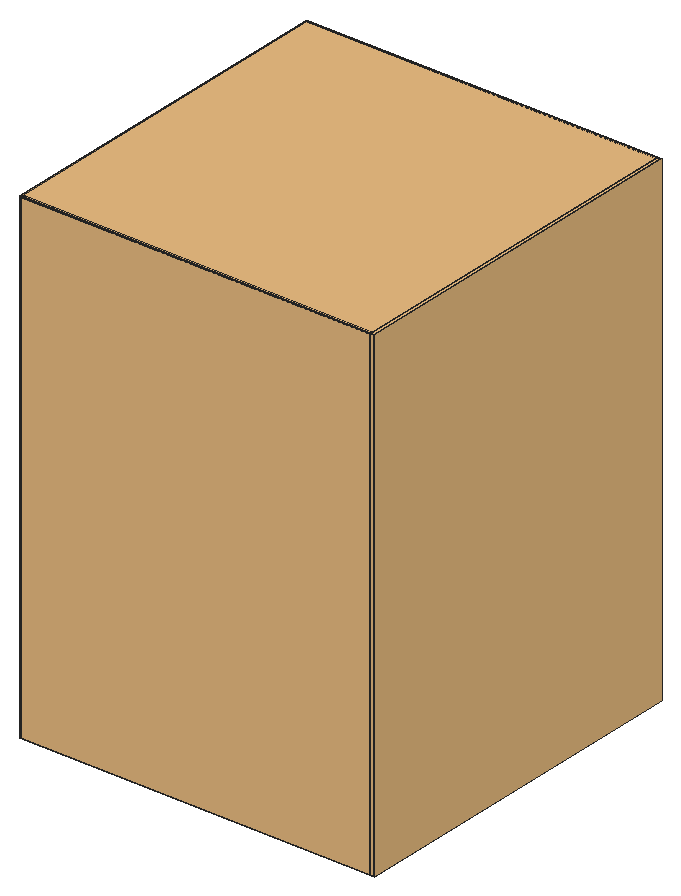
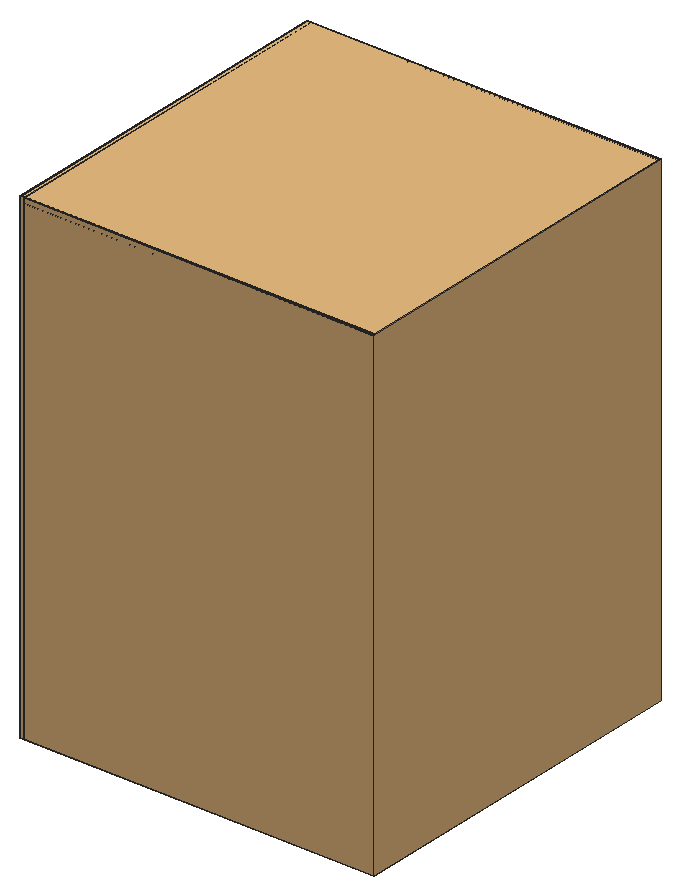
# SketchUp Ruby script. Lengths in inches.
U = 1.inch
M = Sketchup.active_model
def pt(a) = Geom::Point3d.new(a.map { |v| v * U })
def face(e, loops, mat)
  f = e.add_face(loops[0].map { |a| pt(a) })
  loops[1..].each { |l| e.add_face(l.map { |a| pt(a) }).erase! }
  f.material = f.back_material = mat if mat
  f
end
# faces: each face lists its corners as indices into pts; further lists are holes
def faces(e, pts, list, mat = nil) = list.each { |f| face(e, (f[0].is_a?(Array) ? f : [f]).map { |l| l.map { |i| pts[i] } }, mat) }
# xy, xz, yz: faces in a plane at the given z, y or x. An outline is a flat list of corners, or four numbers for a rectangle; further outlines are holes
def ring(l) = l.size == 4 ? [[l[0], l[1]], [l[2], l[1]], [l[2], l[3]], [l[0], l[3]]] : l.each_slice(2).to_a
def flat(e, list, mat, &to3) = list.each { |f| face(e, (f[0].is_a?(Array) ? f : [f]).map { |l| ring(l).map { |u, v| to3.(u, v) } }, mat) }
def xy(e, z, list, mat = nil) = flat(e, list, mat) { |x, y| [x, y, z] }
def xz(e, y, list, mat = nil) = flat(e, list, mat) { |x, z| [x, y, z] }
def yz(e, x, list, mat = nil) = flat(e, list, mat) { |y, z| [x, y, z] }
def lines(e, pts, list) = list.each { |a, b| e.add_line(pt(pts[a]), pt(pts[b])) }
# prism: a flat outline (further loops are holes) pulled along v
def prism(e, loops, v, mat = nil)
  f = face(e, loops, mat); d = Geom::Vector3d.new(v.map { |x| x * U })
  f.pushpull(f.normal.samedirection?(d) ? d.length : -d.length)
end
def box(e, o, s, mat = nil) = prism(e, [[o, [o[0] + s[0], o[1], o[2]], [o[0] + s[0], o[1] + s[1], o[2]], [o[0], o[1] + s[1], o[2]]]], [0, 0, s[2]], mat)
def at(x, y, z, deg = 0) = Geom::Transformation.translation(pt([x, y, z])) * Geom::Transformation.rotation(ORIGIN, Z_AXIS, deg.degrees)
def axes(o, x, y, z) = Geom::Transformation.new([*x, 0, *y, 0, *z, 0, *pt(o).to_a, 1])
def part(name) = M.definitions.add(name)
# library, detail: a bought-in or finely detailed component or shape, given as its bounding box
def library(name, o, s) = part(name).tap { |d| box(d.entities, o, s) }
def detail(e, o, s) = box(e.add_group.entities, o, s)
def put(e, d, t, mat = nil) = e.add_instance(d, t).tap { |i| i.material = mat if mat }
def group(e, t, mat = nil) = e.add_group.tap { |g| g.transformation = t; g.material = mat if mat }.entities
root = M.entities
M.materials.add("green").color = [174, 139, 102]
M.materials.add("vio").color = [206, 114, 100]
c1 = part("3DGeom~220_Defintion")
p = [[-57.64,36.25,-500],[-74.66,-181.39,-451.57],[-284.21,-169.14,-366.97],[199.77,12.4,-463.71],[-284.21,-169.14,-366.97],[-299.61,50.39,-402.32],
  [197.74,223.52,-383.03],[-25.18,244.18,-414.46],[-299.61,50.39,-402.32],[-25.18,244.18,-414.46],[148.26,-202.04,-420.14],[403.65,-14.77,-303.17],
  [374.3125,199.99,-244],[374.3125,199.99,-244],[-71.68,-350.42,-282.14],[-192.66,-343.35,-233.3],[-192.66,-343.35,-233.3],[-284.21,-169.14,-366.97],
  [57.03,-362.35,-264],[324.83,-225.57,-281.11],[-25.18,244.18,-414.46],[-299.61,50.39,-402.32],[-234.73,256.42,-329.86],[142.74,374.75,-199.71],
  [-25.18,244.18,-414.46],[14.03,386.67,-217.86],[-25.18,244.18,-414.46],[-234.73,256.42,-329.86],[142.74,374.75,-199.71],[-25.18,244.18,-414.46],
  [14.03,386.67,-217.86],[-299.61,50.39,-402.32],[-284.21,-169.14,-366.97],[-424.23,-168.6,-189.02],[-461.29,51.02,-196.83],[-234.73,256.42,-329.86],
  [244.68,361.16,-119.44],[374.3125,199.99,-244],[197.74,223.52,-383.03],[197.74,223.52,-383.03],[142.74,374.75,-199.71],[-192.66,-343.35,-233.3],
  [-273.5,-343.04,-130.56],[-234.73,256.42,-329.86],[-374.75,256.97,-151.9],[-106.95,393.74,-169.02],[-374.75,256.97,-151.9],[499.375,-37.98,-61.39],
  [324.83,-225.57,-281.11],[403.65,-14.77,-303.17],[457.21,179.89,-34.61],[403.65,-14.77,-303.17],[403.65,-14.77,-303.17],[374.3125,199.99,-244],
  [-192.66,-343.35,-233.3],[-71.68,-350.42,-282.14],[-49.48,-425.5625,-37.11],[-71.68,-350.42,-282.14],[57.03,-362.35,-264],[158.97,-375.93,-183.73],
  [407.73,-245.68,-71.73],[158.97,-375.93,-183.73],[324.83,-225.57,-281.11],[407.73,-245.68,-71.73],[324.83,-225.57,-281.11],[57.03,-362.35,-264],
  [158.97,-375.93,-183.73],[292.54,349.56,1.44],[374.3125,199.99,-244],[292.54,349.56,1.44],[374.3125,199.99,-244],[244.68,361.16,-119.44],
  [-273.5,-343.04,-130.56],[-192.66,-343.35,-233.3],[49.48,425.5625,37.11],[-457.21,-179.89,34.61],[-499.375,37.98,61.39],[-374.75,256.97,-151.9],
  [-292.54,-349.56,-1.44],[158.97,-375.93,-183.73],[206.83,-387.54,-62.84],[407.73,-245.68,-71.73],[158.97,-375.93,-183.73],[-187.79,394.06,-66.27],
  [-374.75,256.97,-151.9],[-407.73,245.68,71.73],[-407.73,245.68,71.73],[-292.54,-349.56,-1.44],[-273.5,-343.04,-130.56],[292.54,349.56,1.44],
  [374.75,-256.97,151.9],[407.73,-245.68,-71.73],[461.29,-51.02,196.83],[374.75,-256.97,151.9],[-206.83,387.54,62.84],[187.79,-394.06,66.27],
  [374.75,-256.97,151.9],[424.23,168.6,189.02],[-244.68,-361.16,119.44],[-292.54,-349.56,-1.44],[-142.74,-374.75,199.71],[-14.03,-386.67,217.86],
  [106.95,-393.74,169.02],[273.5,343.04,130.56],[273.5,343.04,130.56],[292.54,349.56,1.44],[-244.68,-361.16,119.44],[273.5,343.04,130.56],
  [-244.68,-361.16,119.44],[-374.3125,-199.99,244],[-374.3125,-199.99,244],[192.66,343.35,233.3],[71.68,350.42,282.14],[-57.03,362.35,264],
  [-158.97,375.93,183.73],[-374.3125,-199.99,244],[-403.65,14.77,303.17],[-407.73,245.68,71.73],[-403.65,14.77,303.17],[-324.83,225.57,281.11],
  [-324.83,225.57,281.11],[234.73,-256.42,329.86],[234.73,-256.42,329.86],[374.75,-256.97,151.9],[-407.73,245.68,71.73],[-403.65,14.77,303.17],
  [-324.83,225.57,281.11],[-374.3125,-199.99,244],[192.66,343.35,233.3],[273.5,343.04,130.56],[299.61,-50.39,402.32],[234.73,-256.42,329.86],
  [25.18,-244.18,414.46],[25.18,-244.18,414.46],[234.73,-256.42,329.86],[-158.97,375.93,183.73],[-324.83,225.57,281.11],[-148.26,202.04,420.14],
  [-158.97,375.93,183.73],[-57.03,362.35,264],[284.21,169.14,366.97],[192.66,343.35,233.3],[-197.74,-223.52,383.03],[-142.74,-374.75,199.71],
  [-14.03,-386.67,217.86],[-374.3125,-199.99,244],[-197.74,-223.52,383.03],[-14.03,-386.67,217.86],[25.18,-244.18,414.46],[71.68,350.42,282.14],
  [284.21,169.14,366.97],[192.66,343.35,233.3],[-403.65,14.77,303.17],[-374.3125,-199.99,244],[-57.03,362.35,264],[74.66,181.39,451.57],
  [-57.03,362.35,264],[71.68,350.42,282.14],[-199.77,-12.4,463.71],[71.68,350.42,282.14],[284.21,169.14,366.97],[57.64,-36.25,500],
  [234.73,-256.42,329.86],[234.73,-256.42,329.86],[299.61,-50.39,402.32],[299.61,-50.39,402.32],[284.21,169.14,366.97],[299.61,-50.39,402.32]]
faces(c1.entities,p,[[0,1,2],[3,1,0],[0,4,5],[6,3,0],[7,0,8],[6,0,9],[3,10,1],[11,10,3],
  [12,11,3],[13,3,6],[1,14,15],[10,14,1],[1,16,17],[10,18,14],[19,18,10],[11,19,10],
  [20,21,22],[23,6,24],[25,26,27],[28,29,30],[31,32,33],[31,33,34],[35,31,34],[36,37,38],
  [36,39,40],[32,41,42],[32,42,33],[43,34,44],[45,27,46],[25,27,45],[47,48,49],[50,47,51],
  [50,52,53],[54,55,56],[57,58,56],[19,59,18],[60,61,62],[47,63,64],[65,66,56],[67,50,68],
  [69,70,71],[72,73,56],[40,25,74],[25,45,74],[36,40,74],[34,75,76],[34,33,75],[77,34,76],
  [33,78,75],[33,42,78],[79,80,56],[81,80,82],[45,46,83],[45,83,74],[84,76,85],[83,46,86],
  [87,88,56],[89,36,74],[90,80,91],[92,93,63],[92,63,47],[83,86,94],[83,94,74],[80,95,56],
  [96,95,80],[97,92,47],[97,47,50],[98,99,56],[100,98,56],[101,100,56],[95,102,56],[102,101,56],
  [103,97,50],[104,50,105],[75,78,106],[107,89,74],[75,108,109],[76,75,110],[111,107,74],[112,111,74],
  [113,112,74],[114,113,74],[94,114,74],[76,115,116],[117,76,118],[94,86,119],[94,120,114],[121,102,95],
  [122,95,123],[124,125,126],[127,98,100],[128,97,129],[130,131,93],[130,93,92],[132,101,102],[133,102,134],
  [135,136,137],[138,137,139],[140,92,97],[141,140,97],[140,130,92],[142,143,144],[145,100,146],[142,147,148],
  [149,150,151],[152,153,142],[154,137,155],[156,155,157],[136,152,158],[136,158,137],[159,155,160],[152,142,158],
  [161,148,162],[161,163,164],[155,165,166],[158,142,148],[155,161,167],[158,148,161],[137,158,161],[137,161,155]],"vio")
c2 = library("3DGeom~98_Defintion",[-97.72,-35.49,-500],[195.44,70.98,1000])
c3 = part("3DGeom~99_Defintion")
p = [[97.72,22.79,-497.94],[82.82,12.47,-499.74],[76.21,14.6,-500],[97.72,22.79,-497.94],[76.21,14.6,-500],[71.74,19.25,-499.92],
  [97.72,22.79,-497.94],[71.74,19.25,-499.92],[70.59,25.16,-499.53],[97.72,22.79,-497.94],[89.78,13.42,-499.21],[82.82,12.47,-499.74],
  [97.72,22.79,-497.94],[70.59,25.16,-499.53],[73.07,30.76,-498.92],[97.72,22.79,-497.94],[95.24,17.19,-498.55],[89.78,13.42,-499.21],
  [97.72,22.79,-497.94],[73.07,30.76,-498.92],[78.53,34.54,-498.26],[97.72,22.79,-497.94],[78.53,34.54,-498.26],[85.49,35.49,-497.73],
  [97.72,22.79,-497.94],[85.49,35.49,-497.73],[92.1,33.35,-497.47],[97.72,22.79,-497.94],[92.1,33.35,-497.47],[96.57,28.7,-497.55],
  [-93.36,-33.24,487.31],[-75.65,-25.4,500],[-97.72,-22.56,484.25],[-93.36,-33.24,487.31],[-97.72,-22.56,484.25],[-96.91,-28.5,484.8],
  [-97.72,-22.56,484.25],[-75.65,-25.4,500],[-91.05,-13.3,489.05],[-97.72,-22.56,484.25],[-91.05,-13.3,489.05],[-95.58,-16.99,485.8],
  [-82.33,-34.66,495.19],[-93.36,-33.24,487.31],[-88.02,-35.49,491.12],[-82.33,-34.66,495.19],[-75.65,-25.4,500],[-93.36,-33.24,487.31],
  [-91.05,-13.3,489.05],[-75.65,-25.4,500],[-80.01,-14.72,496.93],[-91.05,-13.3,489.05],[-80.01,-14.72,496.93],[-85.35,-12.47,493.125],
  [-75.65,-25.4,500],[-82.33,-34.66,495.19],[-77.8,-30.96,498.44],[-75.65,-25.4,500],[-76.46,-19.45,499.45],[-80.01,-14.72,496.93]]
faces(c3.entities,p,[[0,1,2],[3,4,5],[6,7,8],[9,10,11],[12,13,14],[15,16,17],[18,19,20],[21,22,23],
  [24,25,26],[27,28,29],[30,31,32],[33,34,35],[36,37,38],[39,40,41],[42,43,44],[45,46,47],
  [48,49,50],[51,52,53],[54,55,56],[57,58,59]],"green")
c4 = part("3DGeom~242_Defintion")
p = [[-230.85,-87.93,-431.85],[22.11,-101.53,-485.51],[16.43,-294.21,-360.73],[264.23,-254.8,-301.01],[16.43,-294.21,-360.73],[269.15,-87.93,-409.08],
  [264.23,-254.8,-301.01],[-231.0625,102.5,-427.26],[21.87,118.36,-480.21],[-230.85,-87.93,-431.85],[268.9375,102.5,-404.49],[-236.35,265.46,-311.23],
  [15.77,306.53,-346.23],[-236.35,265.46,-311.23],[-230.85,-87.93,-431.85],[16.43,-294.21,-360.73],[-235.78,-254.8,-323.78],[-421.96,-50.77,-262.47],
  [-230.85,-87.93,-431.85],[-235.78,-254.8,-323.78],[-422.08,59.18,-259.82],[-230.85,-87.93,-431.85],[-422.08,59.18,-259.82],[-230.85,-87.93,-431.85],
  [-421.96,-50.77,-262.47],[-425.13,153.27,-192.83],[-231.0625,102.5,-427.26],[-422.08,59.18,-259.82],[-236.35,265.46,-311.23],[-231.0625,102.5,-427.26],
  [269.15,-87.93,-409.08],[441.23,-147.11,-160.65],[264.23,-254.8,-301.01],[269.15,-87.93,-409.08],[444.07,-50.76,-223.04],[268.9375,102.5,-404.49],
  [269.15,-87.93,-409.08],[268.9375,102.5,-404.49],[443.95,59.18,-220.39],[263.65,265.47,-288.46],[268.9375,102.5,-404.49],[263.65,265.47,-288.46],
  [-235.78,-254.8,-323.78],[16.43,-294.21,-360.73],[6.34,-408.0625,-139.28],[255.49,-353.39,-109.24],[264.23,-254.8,-301.01],[-245.29,357.3,-114.86],
  [15.77,306.53,-346.23],[-236.35,265.46,-311.23],[5.44,412.57,-119.48],[263.65,265.47,-288.46],[15.77,306.53,-346.23],[-245.29,357.3,-114.86],
  [15.77,306.53,-346.23],[-235.78,-254.8,-323.78],[-244.51,-353.39,-132.01],[-424.8,-147.11,-200.08],[-244.51,-353.39,-132.01],[-430.29,206.29,-79.46],
  [-245.29,357.3,-114.86],[264.23,-254.8,-301.01],[436.18,-204.03,-49.92],[255.49,-353.39,-109.24],[264.23,-254.8,-301.01],[263.65,265.47,-288.46],
  [440.9,153.27,-153.4],[254.71,357.3,-92.09],[263.65,265.47,-288.46],[254.71,357.3,-92.09],[263.65,265.47,-288.46],[-500,0,-22.77],
  [500,0,22.77],[-429.84,-204.03,-89.36],[435.73,206.29,-40.02],[254.71,357.3,-92.09],[-244.51,-353.39,-132.01],[-5.44,-412.57,119.48],
  [245.29,-357.3,114.86],[-244.51,-353.39,-132.01],[-254.71,-357.3,92.09],[-254.71,-357.3,92.09],[-255.49,353.39,109.24],[-6.34,408.0625,139.28],
  [-255.49,353.39,109.24],[-245.29,357.3,-114.86],[-436.18,204.03,49.92],[-255.49,353.39,109.24],[255.49,-353.39,-109.24],[430.29,-206.29,79.46],
  [245.29,-357.3,114.86],[255.49,-353.39,-109.24],[244.51,353.39,132.01],[254.71,357.3,-92.09],[244.51,353.39,132.01],[-435.73,-206.29,40.02],
  [429.84,204.03,89.36],[244.51,353.39,132.01],[-440.9,-153.27,153.4],[-443.95,-59.18,220.39],[-444.07,50.77,223.04],[-441.23,147.11,160.65],
  [425.13,-153.27,192.83],[422.08,-59.18,259.82],[421.96,50.77,262.47],[424.8,147.11,200.08],[-263.65,-265.47,288.46],[245.29,-357.3,114.86],
  [235.78,254.8,323.78],[235.78,254.8,323.78],[244.51,353.39,132.01],[-254.71,-357.3,92.09],[-15.77,-306.53,346.23],[-254.71,-357.3,92.09],
  [-15.77,-306.53,346.23],[-263.65,-265.47,288.46],[-264.22,254.8,301.01],[-264.22,254.8,301.01],[-255.49,353.39,109.24],[236.35,-265.47,311.23],
  [245.29,-357.3,114.86],[236.35,-265.47,311.23],[236.35,-265.47,311.23],[-15.77,-306.53,346.23],[-16.43,294.21,360.73],[235.78,254.8,323.78],
  [-264.22,254.8,301.01],[-268.9375,-102.5,404.49],[236.35,-265.47,311.23],[230.85,87.93,431.85],[230.85,87.93,431.85],[235.78,254.8,323.78],
  [-269.15,87.93,409.08],[236.35,-265.47,311.23],[231.0625,-102.5,427.26],[231.0625,-102.5,427.26],[422.08,-59.18,259.82],[421.96,50.77,262.47],
  [421.96,50.77,262.47],[230.85,87.93,431.85],[-263.65,-265.47,288.46],[-15.77,-306.53,346.23],[-21.87,-118.36,480.21],[-263.65,-265.47,288.46],
  [-268.9375,-102.5,404.49],[-269.15,87.93,409.08],[-16.43,294.21,360.73],[-264.22,254.8,301.01],[236.35,-265.47,311.23],[-22.11,101.53,485.51],
  [235.78,254.8,323.78],[235.78,254.8,323.78],[-16.43,294.21,360.73],[-269.15,87.93,409.08],[-16.43,294.21,360.73],[-268.9375,-102.5,404.49],
  [-268.9375,-102.5,404.49],[-269.15,87.93,409.08]]
faces(c4.entities,p,[[0,1,2],[1,3,4],[1,5,6],[7,8,1],[7,1,9],[8,5,1],[8,10,5],[11,8,7],
  [12,10,8],[13,12,8],[14,15,16],[17,18,19],[20,7,21],[22,23,24],[25,26,27],[25,28,29],
  [30,31,32],[33,34,31],[35,34,36],[37,38,34],[39,38,40],[12,41,10],[42,43,44],[43,45,44],
  [43,46,45],[47,48,49],[50,51,52],[53,50,54],[55,44,56],[57,19,58],[17,19,57],[59,28,25],
  [59,60,28],[61,62,63],[64,31,62],[65,66,38],[67,66,68],[50,69,70],[17,57,71],[27,17,71],
  [25,27,71],[31,34,72],[34,38,72],[38,66,72],[57,58,73],[57,73,71],[59,25,71],[62,31,72],
  [66,74,72],[75,74,66],[76,44,77],[44,78,77],[44,45,78],[79,77,80],[73,58,81],[82,83,50],
  [84,50,85],[83,69,50],[86,87,60],[86,60,59],[88,89,90],[91,62,89],[92,74,93],[83,94,69],
  [73,81,95],[73,95,71],[86,59,71],[89,62,72],[74,96,72],[97,96,74],[95,98,71],[98,99,71],
  [99,100,71],[101,86,71],[100,101,71],[102,89,72],[103,102,72],[104,103,72],[105,104,72],[96,105,72],
  [95,81,106],[95,106,98],[101,87,86],[107,89,102],[108,105,96],[109,96,110],[111,77,112],[113,114,115],
  [101,116,87],[117,83,118],[77,78,119],[120,102,121],[77,122,123],[124,125,94],[124,94,83],[126,124,83],
  [98,106,127],[98,127,99],[100,116,101],[128,102,103],[129,104,105],[130,105,131],[99,127,132],[99,132,100],
  [100,132,116],[133,103,134],[135,136,137],[135,138,139],[140,141,142],[143,142,144],[145,146,147],[141,148,135],
  [149,139,150],[149,151,152],[141,135,142],[153,149,154],[155,142,149],[156,149,157],[142,135,139],[142,139,149]],"vio")
c5 = part("3DGeom~250_Defintion")
p = [[-24.32,49.98,-496.93],[-31.18,-167.76,-459.32],[-244.86,-167.22,-390.18],[228.94,35.96,-443.61],[-244.86,-167.22,-390.18],[-271.06,50.6,-417.1],
  [208.38,242.18,-355.22],[-10.94,254.33,-401.4],[-271.06,50.6,-417.1],[208.38,242.18,-355.22],[-10.94,254.33,-401.4],[-29.68,-340.55,-298.625],
  [-153.05,-340.24,-258.71],[188.15,-179.91,-413.14],[-153.05,-340.24,-258.71],[-244.86,-167.22,-390.18],[420.85,12.3,-271.43],[374.59,221.7,-206.1],
  [374.59,221.7,-206.1],[208.38,242.18,-355.22],[-271.06,50.6,-417.1],[-395.65,-178.42,-224.25],[-445.17,37.67,-225.51],[-244.86,-167.22,-390.18],
  [-224.63,254.87,-332.26],[-10.94,254.33,-401.4],[-271.06,50.6,-417.1],[-224.63,254.87,-332.26],[96.95,-347.5625,-271.96],[354.35,-200.39,-264.02],
  [131.99,383.52,-171.65],[208.38,242.18,-355.22],[-10.94,254.33,-401.4],[5.36,390.53,-198.31],[-224.63,254.87,-332.26],[-240.11,-346.7,-162.91],
  [-153.05,-340.24,-258.71],[227.95,371.69,-85.56],[374.59,221.7,-206.1],[-224.63,254.87,-332.26],[-375.41,243.67,-166.34],[-118.01,390.84,-158.39],
  [-375.41,243.67,-166.34],[-153.05,-340.24,-258.71],[-29.68,-340.55,-298.625],[-20.23,-422.09,-57.92],[-29.68,-340.55,-298.625],[96.95,-347.5625,-271.96],
  [96.95,-347.5625,-271.96],[192.91,-359.39,-185.87],[192.91,-359.39,-185.87],[500,-14.65,-26.51],[354.35,-200.39,-264.02],[420.85,12.3,-271.43],
  [443.13,198.36,6],[420.85,12.3,-271.43],[420.85,12.3,-271.43],[374.59,221.7,-206.1],[422.9,-223.73,-51.92],[192.91,-359.39,-185.87],
  [354.35,-200.39,-264.02],[354.35,-200.39,-264.02],[-240.11,-346.7,-162.91],[-153.05,-340.24,-258.71],[-443.13,-198.36,-6],[-500,14.65,26.51],
  [-267.52,-358.22,-36.9],[267.52,358.22,36.9],[374.59,221.7,-206.1],[267.52,358.22,36.9],[374.59,221.7,-206.1],[227.95,371.69,-85.56],
  [20.23,422.09,57.92],[192.91,-359.39,-185.87],[232.48,-372.86,-63.41],[232.48,-372.86,-63.41],[192.91,-359.39,-185.87],[-422.9,223.73,51.92],
  [-205.0625,384.375,-62.6],[-375.41,243.67,-166.34],[-205.0625,384.375,-62.6],[-267.52,-358.22,-36.9],[-240.11,-346.7,-162.91],[267.52,358.22,36.9],
  [232.48,-372.86,-63.41],[205.0625,-384.375,62.6],[375.41,-243.67,166.34],[205.0625,-384.375,62.6],[-205.0625,384.375,-62.6],[-232.48,372.86,63.41],
  [-232.48,372.86,63.41],[-227.95,-371.69,85.56],[-267.52,-358.22,-36.9],[-131.99,-383.52,171.65],[-227.95,-371.69,85.56],[-5.36,-390.53,198.31],
  [205.0625,-384.375,62.6],[118.01,-390.84,158.39],[445.17,-37.67,225.51],[-227.95,-371.69,85.56],[395.65,178.42,224.25],[-374.59,-221.7,206.1],
  [240.11,346.7,162.91],[240.11,346.7,162.91],[267.52,358.22,36.9],[-420.85,-12.3,271.43],[240.11,346.7,162.91],[-354.35,200.39,264.02],
  [-232.48,372.86,63.41],[153.05,340.24,258.71],[29.68,340.55,298.625],[-96.95,347.5625,271.96],[-192.91,359.39,185.87],[224.63,-254.87,332.26],
  [205.0625,-384.375,62.6],[224.63,-254.87,332.26],[205.0625,-384.375,62.6],[375.41,-243.67,166.34],[-232.48,372.86,63.41],[-192.91,359.39,185.87],
  [-374.59,-221.7,206.1],[-227.95,-371.69,85.56],[10.94,-254.33,401.4],[10.94,-254.33,401.4],[224.63,-254.87,332.26],[153.05,340.24,258.71],
  [240.11,346.7,162.91],[271.0625,-50.61,417.1],[224.63,-254.87,332.26],[-208.38,-242.18,355.22],[-374.59,-221.7,206.1],[-208.38,-242.18,355.22],
  [-192.91,359.39,185.87],[-354.35,200.39,264.02],[-188.15,179.91,413.14],[-192.91,359.39,185.87],[-96.95,347.5625,271.96],[-208.38,-242.18,355.22],
  [10.94,-254.33,401.4],[-420.85,-12.3,271.43],[-374.59,-221.7,206.1],[-208.38,-242.18,355.22],[244.86,167.22,390.18],[153.05,340.24,258.71],
  [29.68,340.55,298.625],[244.86,167.22,390.18],[153.05,340.24,258.71],[-354.35,200.39,264.02],[-420.85,-12.3,271.43],[-228.94,-35.96,443.61],
  [-354.35,200.39,264.02],[-420.85,-12.3,271.43],[-96.95,347.5625,271.96],[31.18,167.76,459.32],[-96.95,347.5625,271.96],[29.68,340.55,298.625],
  [29.68,340.55,298.625],[244.86,167.22,390.18],[24.32,-49.98,496.93],[10.94,-254.33,401.4],[224.63,-254.87,332.26],[224.63,-254.87,332.26],
  [271.0625,-50.61,417.1],[271.0625,-50.61,417.1],[244.86,167.22,390.18],[271.0625,-50.61,417.1]]
faces(c5.entities,p,[[0,1,2],[3,1,0],[0,4,5],[6,3,0],[7,0,8],[9,0,10],[1,11,12],[13,11,1],
  [1,14,15],[3,13,1],[16,13,3],[17,16,3],[18,3,19],[20,21,22],[20,23,21],[24,20,22],
  [25,26,27],[13,28,11],[29,28,13],[16,29,13],[30,31,32],[33,32,34],[30,32,33],[23,35,21],
  [23,36,35],[37,38,31],[37,31,30],[39,22,40],[41,34,42],[33,34,41],[43,44,45],[46,47,45],
  [48,49,45],[29,50,28],[51,52,53],[54,51,55],[54,56,57],[58,59,60],[51,58,61],[62,63,45],
  [22,64,65],[22,21,64],[40,22,65],[21,66,64],[21,35,66],[67,54,68],[69,70,71],[30,33,72],
  [33,41,72],[73,74,45],[58,75,76],[37,30,72],[40,65,77],[78,40,77],[41,79,80],[81,82,45],
  [41,80,72],[83,37,72],[84,85,45],[86,87,75],[86,75,58],[88,77,89],[80,90,72],[91,92,45],
  [93,94,45],[95,93,45],[96,97,45],[97,95,45],[98,86,58],[98,58,51],[64,66,99],[100,98,51],
  [100,51,54],[64,99,101],[65,64,101],[102,100,54],[103,54,104],[65,101,105],[77,65,105],[106,83,72],
  [77,105,107],[108,77,107],[109,106,72],[110,109,72],[111,110,72],[112,111,72],[90,112,72],[113,97,114],
  [115,116,117],[118,107,119],[120,121,93],[122,95,97],[123,97,124],[125,100,126],[127,128,86],[127,86,98],
  [129,93,95],[130,93,131],[132,133,134],[135,134,136],[137,95,138],[139,140,141],[142,98,100],[143,142,100],
  [142,127,98],[144,145,146],[147,148,149],[150,149,134],[151,141,149],[152,134,153],[154,153,155],[156,153,157],
  [158,159,160],[158,161,162],[149,141,159],[153,163,164],[149,159,158],[134,149,158],[134,158,153],[153,158,165]],"vio")
c6 = library("3DGeom~1_Defintion",[-369.63,-500,-363.56],[735.81,1000,728.59])
c7 = library("3DGeom~2_Defintion",[-372.64,-496.69,-369.59],[746.89,1000,738.52])
c8 = library("3DGeom~3_Defintion",[-370.01,-499.5,-356.78],[740.02,1000,722.18])
c9 = library("3DGeom~4_Defintion",[-369.63,-500,-365.03],[739.26,1000,729.3])
c10 = library("3DGeom~5_Defintion",[-370.16,-506.05,-369.45],[742.08,1000,738.24])
c11 = library("3DGeom~6_Defintion",[-367.72,-498.8,-365.91],[735.57,1000,731.94])
g1 = group(root,at(15.3125,38.42,26.21))
put(g1,c1,axes([-2.5,-0.29,7.23],[0,0.00039,0],[0,0,-0.00039],[-0.00039,0,0]),"vio")
g2 = group(root,at(15.3125,38.42,26.21))
put(g2,c2,axes([-1.92,-0.18,7.2],[0,0.00108,0],[0,0,-0.00108],[-0.00108,0,0]),"green")
put(g2,c3,axes([-1.92,-0.18,7.2],[0,0.00108,0],[0,0,-0.00108],[-0.00108,0,0]),"green")
g3 = group(root,at(15.3125,38.42,26.21))
put(g3,c4,axes([-1.86,0.02,7.01],[0,0.00039,0],[0,0,-0.00039],[-0.00039,0,0]),"vio")
g4 = group(root,at(15.3125,38.42,26.21))
put(g4,c5,axes([-1.72,-1.11,7.9375],[0,0.00039,0],[0,0,-0.00039],[-0.00039,0,0]),"vio")
g5 = group(root,at(15.3125,38.42,26.21))
put(g5,c6,axes([-1.67,0,10.71],[0,0.0107,0],[0,0,-0.0107],[-0.0107,0,0]),"green")
put(g5,c7,axes([-1.67,0,10.71],[0,0.01056,0],[0,0,-0.01056],[-0.01056,0,0]),"green")
put(g5,c8,axes([-1.67,0,10.71],[0,0.01069,0],[0,0,-0.01069],[-0.01069,0,0]),"green")
put(g5,c9,axes([-1.67,0,10.71],[0,0.0107,0],[0,0,-0.0107],[-0.0107,0,0]),"green")
put(g5,c10,axes([-1.67,0,10.71],[0,0.01057,0],[0,0,-0.01057],[-0.01057,0,0]),"green")
put(g5,c11,axes([-1.67,0,10.71],[0,0.01067,0],[0,0,-0.01067],[-0.01067,0,0]),"green")
